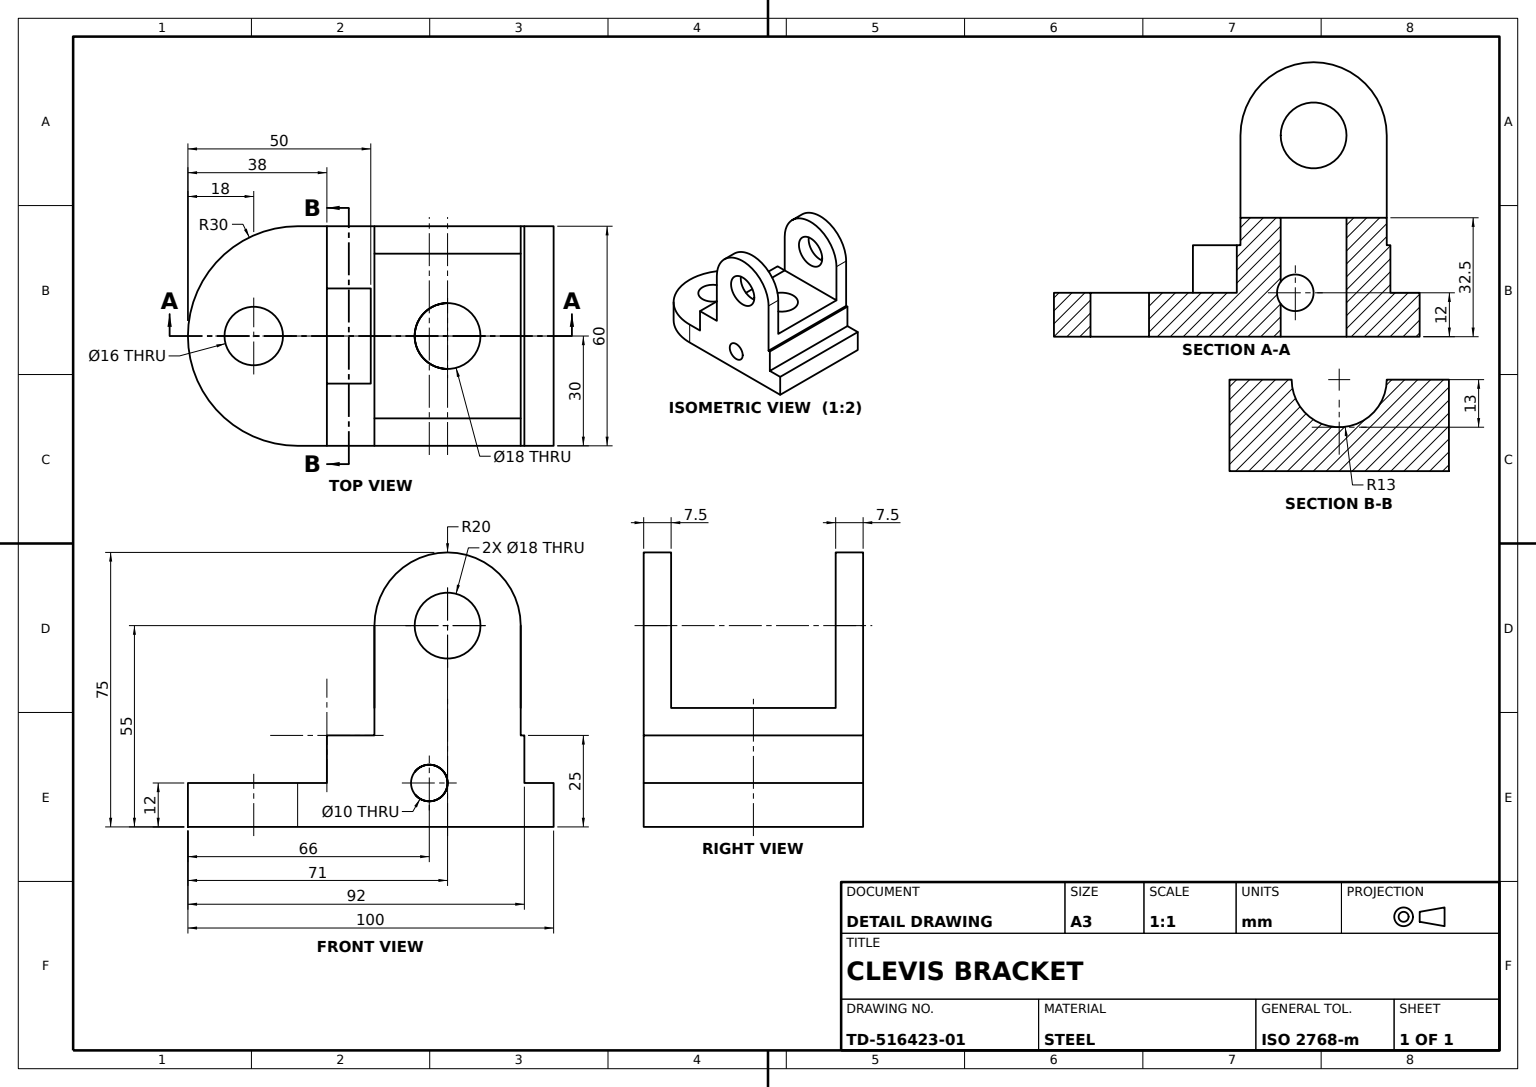
ISO-10303-21;
HEADER;
FILE_DESCRIPTION((''),'2;1');
FILE_NAME('','',(''),(''),'','','');
FILE_SCHEMA(('AUTOMOTIVE_DESIGN'));
ENDSEC;
DATA;
#1=APPLICATION_CONTEXT('');
#2=PRODUCT_CONTEXT('',#1,'mechanical');
#3=PRODUCT('','','',(#2));
#4=PRODUCT_DEFINITION_FORMATION('','',#3);
#5=PRODUCT_DEFINITION_CONTEXT('',#1,'design');
#6=PRODUCT_DEFINITION('','',#4,#5);
#7=PRODUCT_DEFINITION_SHAPE('','',#6);
#8=(LENGTH_UNIT()NAMED_UNIT(*)SI_UNIT(.MILLI.,.METRE.));
#9=(NAMED_UNIT(*)PLANE_ANGLE_UNIT()SI_UNIT($,.RADIAN.));
#10=(NAMED_UNIT(*)SI_UNIT($,.STERADIAN.)SOLID_ANGLE_UNIT());
#11=UNCERTAINTY_MEASURE_WITH_UNIT(LENGTH_MEASURE(1.E-05),#8,'distance_accuracy_value','');
#12=(GEOMETRIC_REPRESENTATION_CONTEXT(3)GLOBAL_UNCERTAINTY_ASSIGNED_CONTEXT((#11))GLOBAL_UNIT_ASSIGNED_CONTEXT((#8,#9,#10))REPRESENTATION_CONTEXT('',''));
#13=CARTESIAN_POINT('',(0.,0.,0.));
#14=VERTEX_POINT('',#13);
#15=CARTESIAN_POINT('',(30.,0.,-30.));
#16=VERTEX_POINT('',#15);
#17=CARTESIAN_POINT('',(0.,0.,-30.));
#18=DIRECTION('',(0.,1.,0.));
#19=DIRECTION('',(0.,0.,1.));
#20=AXIS2_PLACEMENT_3D('',#17,#18,#19);
#21=CIRCLE('',#20,30.);
#22=EDGE_CURVE('',#14,#16,#21,.T.);
#23=ORIENTED_EDGE('',*,*,#22,.T.);
#24=CARTESIAN_POINT('',(30.,12.,-30.));
#25=VERTEX_POINT('',#24);
#26=VECTOR('',#18,1000.);
#27=LINE('',#15,#26);
#28=EDGE_CURVE('',#16,#25,#27,.T.);
#29=ORIENTED_EDGE('',*,*,#28,.T.);
#30=CARTESIAN_POINT('',(0.,12.,0.));
#31=VERTEX_POINT('',#30);
#32=CARTESIAN_POINT('',(0.,12.,-30.));
#33=AXIS2_PLACEMENT_3D('',#32,#18,#19);
#34=CIRCLE('',#33,30.);
#35=EDGE_CURVE('',#31,#25,#34,.T.);
#36=ORIENTED_EDGE('',*,*,#35,.F.);
#37=LINE('',#13,#26);
#38=EDGE_CURVE('',#14,#31,#37,.T.);
#39=ORIENTED_EDGE('',*,*,#38,.F.);
#40=EDGE_LOOP('',(#23,#29,#36,#39));
#41=FACE_OUTER_BOUND('',#40,.T.);
#42=CYLINDRICAL_SURFACE('',#20,30.);
#43=ADVANCED_FACE('',(#41),#42,.T.);
#44=CARTESIAN_POINT('',(-22.5,55.,-51.));
#45=VERTEX_POINT('',#44);
#46=CARTESIAN_POINT('',(-30.,55.,-51.));
#47=VERTEX_POINT('',#46);
#48=DIRECTION('',(-1.,0.,0.));
#49=VECTOR('',#48,1000.);
#50=LINE('',#44,#49);
#51=EDGE_CURVE('',#45,#47,#50,.T.);
#52=ORIENTED_EDGE('',*,*,#51,.F.);
#53=CARTESIAN_POINT('',(-22.5,55.,-91.));
#54=VERTEX_POINT('',#53);
#55=CARTESIAN_POINT('',(-22.5,55.,-71.));
#56=AXIS2_PLACEMENT_3D('',#55,#48,#19);
#57=CIRCLE('',#56,20.);
#58=EDGE_CURVE('',#45,#54,#57,.T.);
#59=ORIENTED_EDGE('',*,*,#58,.T.);
#60=CARTESIAN_POINT('',(-30.,55.,-91.));
#61=VERTEX_POINT('',#60);
#62=LINE('',#53,#49);
#63=EDGE_CURVE('',#54,#61,#62,.T.);
#64=ORIENTED_EDGE('',*,*,#63,.T.);
#65=CARTESIAN_POINT('',(-30.,55.,-71.));
#66=AXIS2_PLACEMENT_3D('',#65,#48,#19);
#67=CIRCLE('',#66,20.);
#68=EDGE_CURVE('',#47,#61,#67,.T.);
#69=ORIENTED_EDGE('',*,*,#68,.F.);
#70=EDGE_LOOP('',(#52,#59,#64,#69));
#71=FACE_OUTER_BOUND('',#70,.T.);
#72=CYLINDRICAL_SURFACE('',#56,20.);
#73=ADVANCED_FACE('',(#71),#72,.T.);
#74=CARTESIAN_POINT('',(-9.,12.,-71.));
#75=VERTEX_POINT('',#74);
#76=CARTESIAN_POINT('',(-30.,12.,-71.));
#77=VERTEX_POINT('',#76);
#78=CARTESIAN_POINT('',(109.,12.,-71.));
#79=LINE('',#78,#49);
#80=EDGE_CURVE('',#75,#77,#79,.T.);
#81=ORIENTED_EDGE('',*,*,#80,.T.);
#82=CARTESIAN_POINT('',(-30.,12.,-61.));
#83=VERTEX_POINT('',#82);
#84=CARTESIAN_POINT('',(-30.,12.,-66.));
#85=AXIS2_PLACEMENT_3D('',#84,#48,#19);
#86=CIRCLE('',#85,5.);
#87=EDGE_CURVE('',#77,#83,#86,.T.);
#88=ORIENTED_EDGE('',*,*,#87,.T.);
#89=CARTESIAN_POINT('',(30.,12.,-61.));
#90=VERTEX_POINT('',#89);
#91=CARTESIAN_POINT('',(109.,12.,-61.));
#92=LINE('',#91,#49);
#93=EDGE_CURVE('',#90,#83,#92,.T.);
#94=ORIENTED_EDGE('',*,*,#93,.F.);
#95=CARTESIAN_POINT('',(30.,12.,-71.));
#96=VERTEX_POINT('',#95);
#97=CARTESIAN_POINT('',(30.,12.,-66.));
#98=AXIS2_PLACEMENT_3D('',#97,#48,#19);
#99=CIRCLE('',#98,5.);
#100=EDGE_CURVE('',#96,#90,#99,.T.);
#101=ORIENTED_EDGE('',*,*,#100,.F.);
#102=CARTESIAN_POINT('',(9.,12.,-71.));
#103=VERTEX_POINT('',#102);
#104=EDGE_CURVE('',#96,#103,#79,.T.);
#105=ORIENTED_EDGE('',*,*,#104,.T.);
#106=CARTESIAN_POINT('',(0.,9.,-62.));
#107=VERTEX_POINT('',#106);
#108=CARTESIAN_POINT('',(0.726741,9.,-62.));
#109=CARTESIAN_POINT('',(1.425372,8.878675,-62.086112));
#110=CARTESIAN_POINT('',(2.78525,8.507616,-62.413297));
#111=CARTESIAN_POINT('',(3.418337,8.271309,-62.647057));
#112=CARTESIAN_POINT('',(4.62738,7.806026,-63.251191));
#113=CARTESIAN_POINT('',(5.207095,7.573243,-63.626891));
#114=CARTESIAN_POINT('',(6.004777,7.296465,-64.287192));
#115=CARTESIAN_POINT('',(6.25998,7.215535,-64.524061));
#116=CARTESIAN_POINT('',(6.748974,7.08685,-65.035396));
#117=CARTESIAN_POINT('',(6.982797,7.039437,-65.310668));
#118=CARTESIAN_POINT('',(7.412294,6.993142,-65.882789));
#119=CARTESIAN_POINT('',(7.610136,6.993459,-66.181706));
#120=CARTESIAN_POINT('',(7.971358,7.055463,-66.806245));
#121=CARTESIAN_POINT('',(8.130031,7.11693,-67.124357));
#122=CARTESIAN_POINT('',(8.333866,7.259246,-67.597621));
#123=CARTESIAN_POINT('',(8.396386,7.315115,-67.755208));
#124=CARTESIAN_POINT('',(8.511134,7.445157,-68.069373));
#125=CARTESIAN_POINT('',(8.56369,7.519975,-68.22709));
#126=CARTESIAN_POINT('',(8.703959,7.769668,-68.688216));
#127=CARTESIAN_POINT('',(8.774291,7.968011,-68.978175));
#128=CARTESIAN_POINT('',(8.854745,8.314584,-69.383685));
#129=CARTESIAN_POINT('',(8.877469,8.439192,-69.51469));
#130=CARTESIAN_POINT('',(8.915274,8.701158,-69.761654));
#131=CARTESIAN_POINT('',(8.930378,8.83809,-69.877421));
#132=CARTESIAN_POINT('',(8.954911,9.123576,-70.093685));
#133=CARTESIAN_POINT('',(8.964335,9.27213,-70.194182));
#134=CARTESIAN_POINT('',(8.979072,9.58097,-70.379581));
#135=CARTESIAN_POINT('',(8.984396,9.742225,-70.46487));
#136=CARTESIAN_POINT('',(8.995994,10.234201,-70.691738));
#137=CARTESIAN_POINT('',(8.998241,10.574237,-70.805941));
#138=CARTESIAN_POINT('',(8.999745,11.10219,-70.922033));
#139=CARTESIAN_POINT('',(8.99989,11.282257,-70.951512));
#140=CARTESIAN_POINT('',(9.000016,11.641387,-70.990393));
#141=CARTESIAN_POINT('',(9.,11.820779,-71.));
#142=B_SPLINE_CURVE_WITH_KNOTS('',3,(#106,#108,#109,#110,#111,#112,#113,#114,#115,#116,#117,#118,#119,#120,#121,#122,#123,#124,#125,#126,#127,#128,#129,#130,#131,#132,#133,#134,#135,#136,#137,#138,#139,#140,#141,#102),.UNSPECIFIED.,.F.,.F.,(4,2,2,2,2,2,2,2,2,2,2,2,2,2,2,2,2,4),(0.,0.002142157,0.004284315,0.006426472,0.007497551,0.00856863,0.009639708,0.010710787,0.011246327,0.011781866,0.012852945,0.013388484,0.013924023,0.014459563,0.014995102,0.016066181,0.01660172,0.01713726),.UNSPECIFIED.);
#143=EDGE_CURVE('',#107,#103,#142,.T.);
#144=ORIENTED_EDGE('',*,*,#143,.F.);
#145=CARTESIAN_POINT('',(-9.,11.8209,-71.));
#146=CARTESIAN_POINT('',(-9.000016,11.641774,-70.990405));
#147=CARTESIAN_POINT('',(-8.999891,11.283468,-70.951672));
#148=CARTESIAN_POINT('',(-8.999747,11.103386,-70.922255));
#149=CARTESIAN_POINT('',(-8.998246,10.575033,-70.806197));
#150=CARTESIAN_POINT('',(-8.995995,10.235538,-70.692133));
#151=CARTESIAN_POINT('',(-8.984485,9.745344,-70.466417));
#152=CARTESIAN_POINT('',(-8.979195,9.584172,-70.381362));
#153=CARTESIAN_POINT('',(-8.964482,9.274613,-70.195811));
#154=CARTESIAN_POINT('',(-8.955082,9.126074,-70.095418));
#155=CARTESIAN_POINT('',(-8.93069,8.841205,-69.879937));
#156=CARTESIAN_POINT('',(-8.915701,8.704875,-69.764847));
#157=CARTESIAN_POINT('',(-8.878347,8.444548,-69.520041));
#158=CARTESIAN_POINT('',(-8.855808,8.319832,-69.389454));
#159=CARTESIAN_POINT('',(-8.775159,7.970443,-68.981745));
#160=CARTESIAN_POINT('',(-8.704837,7.772204,-68.691882));
#161=CARTESIAN_POINT('',(-8.519744,7.440793,-68.081856));
#162=CARTESIAN_POINT('',(-8.403721,7.308286,-67.760082));
#163=CARTESIAN_POINT('',(-8.198666,7.164719,-67.283581));
#164=CARTESIAN_POINT('',(-8.124892,7.125469,-67.124746));
#165=CARTESIAN_POINT('',(-7.965912,7.063018,-66.807662));
#166=CARTESIAN_POINT('',(-7.880201,7.03977,-66.648579));
#167=CARTESIAN_POINT('',(-7.609601,6.99346,-66.1809));
#168=CARTESIAN_POINT('',(-7.411303,6.993087,-65.881207));
#169=CARTESIAN_POINT('',(-6.979026,7.040007,-65.305911));
#170=CARTESIAN_POINT('',(-6.745093,7.087759,-65.031095));
#171=CARTESIAN_POINT('',(-6.257885,7.216199,-64.522116));
#172=CARTESIAN_POINT('',(-6.002691,7.29713,-64.285268));
#173=CARTESIAN_POINT('',(-5.468957,7.482442,-63.843853));
#174=CARTESIAN_POINT('',(-5.188651,7.587613,-63.638291));
#175=CARTESIAN_POINT('',(-4.61524,7.808165,-63.265892));
#176=CARTESIAN_POINT('',(-4.321594,7.92372,-63.098261));
#177=CARTESIAN_POINT('',(-3.718366,8.15583,-62.79711));
#178=CARTESIAN_POINT('',(-3.408815,8.272473,-62.663595));
#179=CARTESIAN_POINT('',(-2.769917,8.495453,-62.430097));
#180=CARTESIAN_POINT('',(-2.437965,8.602548,-62.329528));
#181=CARTESIAN_POINT('',(-1.762154,8.786606,-62.167358));
#182=CARTESIAN_POINT('',(-1.419129,8.863377,-62.10562));
#183=CARTESIAN_POINT('',(-0.720045,8.970201,-62.021945));
#184=CARTESIAN_POINT('',(-0.362595,9.,-62.));
#185=B_SPLINE_CURVE_WITH_KNOTS('',3,(#74,#145,#146,#147,#148,#149,#150,#151,#152,#153,#154,#155,#156,#157,#158,#159,#160,#161,#162,#163,#164,#165,#166,#167,#168,#169,#170,#171,#172,#173,#174,#175,#176,#177,#178,#179,#180,#181,#182,#183,#184,#106),.UNSPECIFIED.,.F.,.F.,(4,2,2,2,2,2,2,2,2,2,2,2,2,2,2,2,2,2,2,2,4),(0.051380768,0.051915165,0.052449561,0.053518354,0.054052751,0.054587147,0.055121544,0.05565594,0.056724733,0.057793526,0.058327923,0.058862319,0.059931112,0.060999905,0.062068698,0.063137491,0.064206284,0.065275077,0.06634387,0.067412663,0.068481455),.UNSPECIFIED.);
#186=EDGE_CURVE('',#75,#107,#185,.T.);
#187=ORIENTED_EDGE('',*,*,#186,.F.);
#188=EDGE_LOOP('',(#81,#88,#94,#101,#105,#144,#187));
#189=FACE_OUTER_BOUND('',#188,.T.);
#190=CARTESIAN_POINT('',(109.,12.,-66.));
#191=AXIS2_PLACEMENT_3D('',#190,#48,#19);
#192=CYLINDRICAL_SURFACE('',#191,5.);
#193=ADVANCED_FACE('',(#189),#192,.F.);
#194=CARTESIAN_POINT('',(0.,12.,-38.));
#195=VERTEX_POINT('',#194);
#196=CARTESIAN_POINT('',(13.,25.,-38.));
#197=VERTEX_POINT('',#196);
#198=CARTESIAN_POINT('',(0.,25.,-38.));
#199=DIRECTION('',(1.,0.,0.));
#200=AXIS2_PLACEMENT_3D('',#198,#19,#199);
#201=CIRCLE('',#200,13.);
#202=EDGE_CURVE('',#195,#197,#201,.T.);
#203=ORIENTED_EDGE('',*,*,#202,.F.);
#204=CARTESIAN_POINT('',(30.,12.,-38.));
#205=VERTEX_POINT('',#204);
#206=CARTESIAN_POINT('',(-30.,12.,-38.));
#207=VECTOR('',#199,1000.);
#208=LINE('',#206,#207);
#209=EDGE_CURVE('',#195,#205,#208,.T.);
#210=ORIENTED_EDGE('',*,*,#209,.T.);
#211=CARTESIAN_POINT('',(30.,25.,-38.));
#212=VERTEX_POINT('',#211);
#213=DIRECTION('',(0.,-1.,0.));
#214=VECTOR('',#213,1000.);
#215=LINE('',#204,#214);
#216=EDGE_CURVE('',#212,#205,#215,.T.);
#217=ORIENTED_EDGE('',*,*,#216,.F.);
#218=CARTESIAN_POINT('',(-30.,25.,-38.));
#219=LINE('',#218,#207);
#220=EDGE_CURVE('',#197,#212,#219,.T.);
#221=ORIENTED_EDGE('',*,*,#220,.F.);
#222=EDGE_LOOP('',(#203,#210,#217,#221));
#223=FACE_OUTER_BOUND('',#222,.T.);
#224=AXIS2_PLACEMENT_3D('',#206,#19,#199);
#225=PLANE('',#224);
#226=ADVANCED_FACE('',(#223),#225,.T.);
#227=CARTESIAN_POINT('',(30.,12.,-100.));
#228=VERTEX_POINT('',#227);
#229=CARTESIAN_POINT('',(-30.,12.,-100.));
#230=VERTEX_POINT('',#229);
#231=LINE('',#229,#49);
#232=EDGE_CURVE('',#228,#230,#231,.T.);
#233=ORIENTED_EDGE('',*,*,#232,.F.);
#234=CARTESIAN_POINT('',(30.,0.,-100.));
#235=VERTEX_POINT('',#234);
#236=LINE('',#227,#214);
#237=EDGE_CURVE('',#228,#235,#236,.T.);
#238=ORIENTED_EDGE('',*,*,#237,.T.);
#239=CARTESIAN_POINT('',(-30.,0.,-100.));
#240=VERTEX_POINT('',#239);
#241=LINE('',#239,#49);
#242=EDGE_CURVE('',#235,#240,#241,.T.);
#243=ORIENTED_EDGE('',*,*,#242,.T.);
#244=LINE('',#229,#214);
#245=EDGE_CURVE('',#230,#240,#244,.T.);
#246=ORIENTED_EDGE('',*,*,#245,.F.);
#247=EDGE_LOOP('',(#233,#238,#243,#246));
#248=FACE_OUTER_BOUND('',#247,.T.);
#249=AXIS2_PLACEMENT_3D('',#229,#19,#199);
#250=PLANE('',#249);
#251=ADVANCED_FACE('',(#248),#250,.F.);
#252=CARTESIAN_POINT('',(-30.,25.,-91.));
#253=VERTEX_POINT('',#252);
#254=CARTESIAN_POINT('',(-30.,25.,-92.));
#255=VERTEX_POINT('',#254);
#256=CARTESIAN_POINT('',(-30.,25.,0.));
#257=DIRECTION('',(0.,0.,-1.));
#258=VECTOR('',#257,1000.);
#259=LINE('',#256,#258);
#260=EDGE_CURVE('',#253,#255,#259,.T.);
#261=ORIENTED_EDGE('',*,*,#260,.F.);
#262=CARTESIAN_POINT('',(30.,25.,-91.));
#263=VERTEX_POINT('',#262);
#264=CARTESIAN_POINT('',(-22.5,25.,-91.));
#265=LINE('',#264,#49);
#266=EDGE_CURVE('',#263,#253,#265,.T.);
#267=ORIENTED_EDGE('',*,*,#266,.F.);
#268=CARTESIAN_POINT('',(30.,25.,-92.));
#269=VERTEX_POINT('',#268);
#270=CARTESIAN_POINT('',(30.,25.,0.));
#271=LINE('',#270,#258);
#272=EDGE_CURVE('',#263,#269,#271,.T.);
#273=ORIENTED_EDGE('',*,*,#272,.T.);
#274=LINE('',#254,#207);
#275=EDGE_CURVE('',#255,#269,#274,.T.);
#276=ORIENTED_EDGE('',*,*,#275,.F.);
#277=EDGE_LOOP('',(#261,#267,#273,#276));
#278=FACE_OUTER_BOUND('',#277,.T.);
#279=AXIS2_PLACEMENT_3D('',#256,#213,#257);
#280=PLANE('',#279);
#281=ADVANCED_FACE('',(#278),#280,.F.);
#282=CARTESIAN_POINT('',(22.5,55.,-51.));
#283=VERTEX_POINT('',#282);
#284=CARTESIAN_POINT('',(30.,55.,-51.));
#285=VERTEX_POINT('',#284);
#286=LINE('',#282,#207);
#287=EDGE_CURVE('',#283,#285,#286,.T.);
#288=ORIENTED_EDGE('',*,*,#287,.F.);
#289=CARTESIAN_POINT('',(22.5,32.5,-51.));
#290=VERTEX_POINT('',#289);
#291=LINE('',#282,#26);
#292=EDGE_CURVE('',#290,#283,#291,.T.);
#293=ORIENTED_EDGE('',*,*,#292,.F.);
#294=CARTESIAN_POINT('',(-22.5,32.5,-51.));
#295=VERTEX_POINT('',#294);
#296=LINE('',#294,#207);
#297=EDGE_CURVE('',#295,#290,#296,.T.);
#298=ORIENTED_EDGE('',*,*,#297,.F.);
#299=LINE('',#44,#26);
#300=EDGE_CURVE('',#295,#45,#299,.T.);
#301=ORIENTED_EDGE('',*,*,#300,.T.);
#302=ORIENTED_EDGE('',*,*,#51,.T.);
#303=CARTESIAN_POINT('',(-30.,25.,-51.));
#304=VERTEX_POINT('',#303);
#305=LINE('',#46,#26);
#306=EDGE_CURVE('',#304,#47,#305,.T.);
#307=ORIENTED_EDGE('',*,*,#306,.F.);
#308=CARTESIAN_POINT('',(30.,25.,-51.));
#309=VERTEX_POINT('',#308);
#310=CARTESIAN_POINT('',(-22.5,25.,-51.));
#311=LINE('',#310,#49);
#312=EDGE_CURVE('',#309,#304,#311,.T.);
#313=ORIENTED_EDGE('',*,*,#312,.F.);
#314=LINE('',#284,#26);
#315=EDGE_CURVE('',#309,#285,#314,.T.);
#316=ORIENTED_EDGE('',*,*,#315,.T.);
#317=EDGE_LOOP('',(#288,#293,#298,#301,#302,#307,#313,#316));
#318=FACE_OUTER_BOUND('',#317,.T.);
#319=AXIS2_PLACEMENT_3D('',#44,#19,#199);
#320=PLANE('',#319);
#321=ADVANCED_FACE('',(#318),#320,.T.);
#322=CARTESIAN_POINT('',(-30.,0.,-30.));
#323=VERTEX_POINT('',#322);
#324=CARTESIAN_POINT('',(-30.,12.,-30.));
#325=VERTEX_POINT('',#324);
#326=LINE('',#322,#26);
#327=EDGE_CURVE('',#323,#325,#326,.T.);
#328=ORIENTED_EDGE('',*,*,#327,.F.);
#329=EDGE_CURVE('',#323,#14,#21,.T.);
#330=ORIENTED_EDGE('',*,*,#329,.T.);
#331=ORIENTED_EDGE('',*,*,#38,.T.);
#332=EDGE_CURVE('',#325,#31,#34,.T.);
#333=ORIENTED_EDGE('',*,*,#332,.F.);
#334=EDGE_LOOP('',(#328,#330,#331,#333));
#335=FACE_OUTER_BOUND('',#334,.T.);
#336=ADVANCED_FACE('',(#335),#42,.T.);
#337=CARTESIAN_POINT('',(30.,12.,-92.));
#338=VERTEX_POINT('',#337);
#339=LINE('',#227,#258);
#340=EDGE_CURVE('',#338,#228,#339,.T.);
#341=ORIENTED_EDGE('',*,*,#340,.T.);
#342=ORIENTED_EDGE('',*,*,#232,.T.);
#343=CARTESIAN_POINT('',(-30.,12.,-92.));
#344=VERTEX_POINT('',#343);
#345=CARTESIAN_POINT('',(-30.,12.,0.));
#346=VECTOR('',#19,1000.);
#347=LINE('',#345,#346);
#348=EDGE_CURVE('',#230,#344,#347,.T.);
#349=ORIENTED_EDGE('',*,*,#348,.T.);
#350=CARTESIAN_POINT('',(0.,12.,-92.));
#351=LINE('',#350,#49);
#352=EDGE_CURVE('',#338,#344,#351,.T.);
#353=ORIENTED_EDGE('',*,*,#352,.F.);
#354=EDGE_LOOP('',(#341,#342,#349,#353));
#355=FACE_OUTER_BOUND('',#354,.T.);
#356=AXIS2_PLACEMENT_3D('',#30,#213,#257);
#357=PLANE('',#356);
#358=ADVANCED_FACE('',(#355),#357,.F.);
#359=CARTESIAN_POINT('',(-22.5,55.,-62.));
#360=VERTEX_POINT('',#359);
#361=CARTESIAN_POINT('',(-30.,55.,-62.));
#362=VERTEX_POINT('',#361);
#363=CARTESIAN_POINT('',(109.,55.,-62.));
#364=LINE('',#363,#49);
#365=EDGE_CURVE('',#360,#362,#364,.T.);
#366=ORIENTED_EDGE('',*,*,#365,.F.);
#367=CARTESIAN_POINT('',(-22.5,55.,-80.));
#368=VERTEX_POINT('',#367);
#369=CIRCLE('',#56,9.);
#370=EDGE_CURVE('',#368,#360,#369,.T.);
#371=ORIENTED_EDGE('',*,*,#370,.F.);
#372=CARTESIAN_POINT('',(-30.,55.,-80.));
#373=VERTEX_POINT('',#372);
#374=CARTESIAN_POINT('',(109.,55.,-80.));
#375=LINE('',#374,#49);
#376=EDGE_CURVE('',#368,#373,#375,.T.);
#377=ORIENTED_EDGE('',*,*,#376,.T.);
#378=CIRCLE('',#66,9.);
#379=EDGE_CURVE('',#373,#362,#378,.T.);
#380=ORIENTED_EDGE('',*,*,#379,.T.);
#381=EDGE_LOOP('',(#366,#371,#377,#380));
#382=FACE_OUTER_BOUND('',#381,.T.);
#383=CARTESIAN_POINT('',(109.,55.,-71.));
#384=AXIS2_PLACEMENT_3D('',#383,#48,#19);
#385=CYLINDRICAL_SURFACE('',#384,9.);
#386=ADVANCED_FACE('',(#382),#385,.F.);
#387=CARTESIAN_POINT('',(0.,0.,-10.));
#388=VERTEX_POINT('',#387);
#389=CARTESIAN_POINT('',(0.,0.,-26.));
#390=VERTEX_POINT('',#389);
#391=CARTESIAN_POINT('',(0.,0.,-18.));
#392=AXIS2_PLACEMENT_3D('',#391,#213,#257);
#393=CIRCLE('',#392,8.);
#394=EDGE_CURVE('',#388,#390,#393,.T.);
#395=ORIENTED_EDGE('',*,*,#394,.T.);
#396=CARTESIAN_POINT('',(0.,12.,-26.));
#397=VERTEX_POINT('',#396);
#398=CARTESIAN_POINT('',(0.,-127.,-26.));
#399=LINE('',#398,#26);
#400=EDGE_CURVE('',#390,#397,#399,.T.);
#401=ORIENTED_EDGE('',*,*,#400,.T.);
#402=CARTESIAN_POINT('',(0.,12.,-10.));
#403=VERTEX_POINT('',#402);
#404=CARTESIAN_POINT('',(0.,12.,-18.));
#405=AXIS2_PLACEMENT_3D('',#404,#18,#19);
#406=CIRCLE('',#405,8.);
#407=EDGE_CURVE('',#397,#403,#406,.T.);
#408=ORIENTED_EDGE('',*,*,#407,.T.);
#409=CARTESIAN_POINT('',(0.,-127.,-10.));
#410=LINE('',#409,#26);
#411=EDGE_CURVE('',#388,#403,#410,.T.);
#412=ORIENTED_EDGE('',*,*,#411,.F.);
#413=EDGE_LOOP('',(#395,#401,#408,#412));
#414=FACE_OUTER_BOUND('',#413,.T.);
#415=CARTESIAN_POINT('',(0.,-127.,-18.));
#416=AXIS2_PLACEMENT_3D('',#415,#18,#19);
#417=CYLINDRICAL_SURFACE('',#416,8.);
#418=ADVANCED_FACE('',(#414),#417,.F.);
#419=ORIENTED_EDGE('',*,*,#352,.T.);
#420=CARTESIAN_POINT('',(-30.,0.,-92.));
#421=LINE('',#420,#214);
#422=EDGE_CURVE('',#255,#344,#421,.T.);
#423=ORIENTED_EDGE('',*,*,#422,.F.);
#424=ORIENTED_EDGE('',*,*,#275,.T.);
#425=CARTESIAN_POINT('',(30.,0.,-92.));
#426=LINE('',#425,#214);
#427=EDGE_CURVE('',#269,#338,#426,.T.);
#428=ORIENTED_EDGE('',*,*,#427,.T.);
#429=EDGE_LOOP('',(#419,#423,#424,#428));
#430=FACE_OUTER_BOUND('',#429,.T.);
#431=AXIS2_PLACEMENT_3D('',#420,#19,#199);
#432=PLANE('',#431);
#433=ADVANCED_FACE('',(#430),#432,.F.);
#434=EDGE_CURVE('',#403,#397,#406,.T.);
#435=ORIENTED_EDGE('',*,*,#434,.T.);
#436=ORIENTED_EDGE('',*,*,#400,.F.);
#437=EDGE_CURVE('',#390,#388,#393,.T.);
#438=ORIENTED_EDGE('',*,*,#437,.T.);
#439=ORIENTED_EDGE('',*,*,#411,.T.);
#440=EDGE_LOOP('',(#435,#436,#438,#439));
#441=FACE_OUTER_BOUND('',#440,.T.);
#442=ADVANCED_FACE('',(#441),#417,.F.);
#443=ORIENTED_EDGE('',*,*,#370,.T.);
#444=EDGE_CURVE('',#360,#368,#369,.T.);
#445=ORIENTED_EDGE('',*,*,#444,.T.);
#446=EDGE_LOOP('',(#443,#445));
#447=FACE_BOUND('',#446,.T.);
#448=CARTESIAN_POINT('',(-22.5,32.5,-91.));
#449=VERTEX_POINT('',#448);
#450=LINE('',#264,#214);
#451=EDGE_CURVE('',#54,#449,#450,.T.);
#452=ORIENTED_EDGE('',*,*,#451,.F.);
#453=ORIENTED_EDGE('',*,*,#58,.F.);
#454=ORIENTED_EDGE('',*,*,#300,.F.);
#455=LINE('',#448,#346);
#456=EDGE_CURVE('',#449,#295,#455,.T.);
#457=ORIENTED_EDGE('',*,*,#456,.F.);
#458=EDGE_LOOP('',(#452,#453,#454,#457));
#459=FACE_OUTER_BOUND('',#458,.T.);
#460=PLANE('',#56);
#461=ADVANCED_FACE('',(#447,#459),#460,.F.);
#462=ORIENTED_EDGE('',*,*,#100,.T.);
#463=EDGE_CURVE('',#90,#96,#99,.T.);
#464=ORIENTED_EDGE('',*,*,#463,.T.);
#465=EDGE_LOOP('',(#462,#464));
#466=FACE_BOUND('',#465,.T.);
#467=CARTESIAN_POINT('',(30.,55.,-62.));
#468=VERTEX_POINT('',#467);
#469=CARTESIAN_POINT('',(30.,55.,-80.));
#470=VERTEX_POINT('',#469);
#471=CARTESIAN_POINT('',(30.,55.,-71.));
#472=AXIS2_PLACEMENT_3D('',#471,#48,#19);
#473=CIRCLE('',#472,9.);
#474=EDGE_CURVE('',#468,#470,#473,.T.);
#475=ORIENTED_EDGE('',*,*,#474,.T.);
#476=EDGE_CURVE('',#470,#468,#473,.T.);
#477=ORIENTED_EDGE('',*,*,#476,.T.);
#478=EDGE_LOOP('',(#475,#477));
#479=FACE_BOUND('',#478,.T.);
#480=EDGE_CURVE('',#212,#309,#271,.T.);
#481=ORIENTED_EDGE('',*,*,#480,.F.);
#482=ORIENTED_EDGE('',*,*,#216,.T.);
#483=EDGE_CURVE('',#25,#205,#339,.T.);
#484=ORIENTED_EDGE('',*,*,#483,.F.);
#485=ORIENTED_EDGE('',*,*,#28,.F.);
#486=LINE('',#234,#258);
#487=EDGE_CURVE('',#16,#235,#486,.T.);
#488=ORIENTED_EDGE('',*,*,#487,.T.);
#489=ORIENTED_EDGE('',*,*,#237,.F.);
#490=ORIENTED_EDGE('',*,*,#340,.F.);
#491=ORIENTED_EDGE('',*,*,#427,.F.);
#492=ORIENTED_EDGE('',*,*,#272,.F.);
#493=CARTESIAN_POINT('',(30.,55.,-91.));
#494=VERTEX_POINT('',#493);
#495=LINE('',#262,#214);
#496=EDGE_CURVE('',#494,#263,#495,.T.);
#497=ORIENTED_EDGE('',*,*,#496,.F.);
#498=CIRCLE('',#472,20.);
#499=EDGE_CURVE('',#285,#494,#498,.T.);
#500=ORIENTED_EDGE('',*,*,#499,.F.);
#501=ORIENTED_EDGE('',*,*,#315,.F.);
#502=EDGE_LOOP('',(#481,#482,#484,#485,#488,#489,#490,#491,#492,#497,#500,#501));
#503=FACE_OUTER_BOUND('',#502,.T.);
#504=AXIS2_PLACEMENT_3D('',#227,#48,#19);
#505=PLANE('',#504);
#506=ADVANCED_FACE('',(#466,#479,#503),#505,.F.);
#507=ORIENTED_EDGE('',*,*,#407,.F.);
#508=ORIENTED_EDGE('',*,*,#434,.F.);
#509=EDGE_LOOP('',(#507,#508));
#510=FACE_BOUND('',#509,.T.);
#511=ORIENTED_EDGE('',*,*,#35,.T.);
#512=ORIENTED_EDGE('',*,*,#483,.T.);
#513=ORIENTED_EDGE('',*,*,#209,.F.);
#514=VERTEX_POINT('',#206);
#515=EDGE_CURVE('',#514,#195,#208,.T.);
#516=ORIENTED_EDGE('',*,*,#515,.F.);
#517=EDGE_CURVE('',#514,#325,#347,.T.);
#518=ORIENTED_EDGE('',*,*,#517,.T.);
#519=ORIENTED_EDGE('',*,*,#332,.T.);
#520=EDGE_LOOP('',(#511,#512,#513,#516,#518,#519));
#521=FACE_OUTER_BOUND('',#520,.T.);
#522=ADVANCED_FACE('',(#510,#521),#357,.F.);
#523=ORIENTED_EDGE('',*,*,#476,.F.);
#524=CARTESIAN_POINT('',(22.5,55.,-80.));
#525=VERTEX_POINT('',#524);
#526=EDGE_CURVE('',#470,#525,#375,.T.);
#527=ORIENTED_EDGE('',*,*,#526,.T.);
#528=CARTESIAN_POINT('',(22.5,55.,-62.));
#529=VERTEX_POINT('',#528);
#530=CARTESIAN_POINT('',(22.5,55.,-71.));
#531=AXIS2_PLACEMENT_3D('',#530,#199,#257);
#532=CIRCLE('',#531,9.);
#533=EDGE_CURVE('',#529,#525,#532,.T.);
#534=ORIENTED_EDGE('',*,*,#533,.F.);
#535=EDGE_CURVE('',#468,#529,#364,.T.);
#536=ORIENTED_EDGE('',*,*,#535,.F.);
#537=EDGE_LOOP('',(#523,#527,#534,#536));
#538=FACE_OUTER_BOUND('',#537,.T.);
#539=ADVANCED_FACE('',(#538),#385,.F.);
#540=CARTESIAN_POINT('',(22.5,32.5,-91.));
#541=VERTEX_POINT('',#540);
#542=LINE('',#289,#258);
#543=EDGE_CURVE('',#290,#541,#542,.T.);
#544=ORIENTED_EDGE('',*,*,#543,.T.);
#545=LINE('',#540,#49);
#546=EDGE_CURVE('',#541,#449,#545,.T.);
#547=ORIENTED_EDGE('',*,*,#546,.T.);
#548=ORIENTED_EDGE('',*,*,#456,.T.);
#549=ORIENTED_EDGE('',*,*,#297,.T.);
#550=EDGE_LOOP('',(#544,#547,#548,#549));
#551=FACE_OUTER_BOUND('',#550,.T.);
#552=CARTESIAN_POINT('',(0.,32.5,-80.));
#553=VERTEX_POINT('',#552);
#554=CARTESIAN_POINT('',(0.,32.5,-62.));
#555=VERTEX_POINT('',#554);
#556=CARTESIAN_POINT('',(0.,32.5,-71.));
#557=AXIS2_PLACEMENT_3D('',#556,#18,#19);
#558=CIRCLE('',#557,9.);
#559=EDGE_CURVE('',#553,#555,#558,.T.);
#560=ORIENTED_EDGE('',*,*,#559,.F.);
#561=EDGE_CURVE('',#555,#553,#558,.T.);
#562=ORIENTED_EDGE('',*,*,#561,.F.);
#563=EDGE_LOOP('',(#560,#562));
#564=FACE_BOUND('',#563,.T.);
#565=CARTESIAN_POINT('',(0.,32.5,0.));
#566=AXIS2_PLACEMENT_3D('',#565,#18,#19);
#567=PLANE('',#566);
#568=ADVANCED_FACE('',(#551,#564),#567,.T.);
#569=VERTEX_POINT('',#218);
#570=CARTESIAN_POINT('',(-13.,25.,-38.));
#571=VERTEX_POINT('',#570);
#572=EDGE_CURVE('',#569,#571,#219,.T.);
#573=ORIENTED_EDGE('',*,*,#572,.F.);
#574=LINE('',#206,#214);
#575=EDGE_CURVE('',#569,#514,#574,.T.);
#576=ORIENTED_EDGE('',*,*,#575,.T.);
#577=ORIENTED_EDGE('',*,*,#515,.T.);
#578=EDGE_CURVE('',#571,#195,#201,.T.);
#579=ORIENTED_EDGE('',*,*,#578,.F.);
#580=EDGE_LOOP('',(#573,#576,#577,#579));
#581=FACE_OUTER_BOUND('',#580,.T.);
#582=ADVANCED_FACE('',(#581),#225,.T.);
#583=ORIENTED_EDGE('',*,*,#496,.T.);
#584=ORIENTED_EDGE('',*,*,#266,.T.);
#585=LINE('',#252,#214);
#586=EDGE_CURVE('',#61,#253,#585,.T.);
#587=ORIENTED_EDGE('',*,*,#586,.F.);
#588=ORIENTED_EDGE('',*,*,#63,.F.);
#589=ORIENTED_EDGE('',*,*,#451,.T.);
#590=ORIENTED_EDGE('',*,*,#546,.F.);
#591=CARTESIAN_POINT('',(22.5,55.,-91.));
#592=VERTEX_POINT('',#591);
#593=CARTESIAN_POINT('',(22.5,25.,-91.));
#594=LINE('',#593,#214);
#595=EDGE_CURVE('',#592,#541,#594,.T.);
#596=ORIENTED_EDGE('',*,*,#595,.F.);
#597=LINE('',#591,#207);
#598=EDGE_CURVE('',#592,#494,#597,.T.);
#599=ORIENTED_EDGE('',*,*,#598,.T.);
#600=EDGE_LOOP('',(#583,#584,#587,#588,#589,#590,#596,#599));
#601=FACE_OUTER_BOUND('',#600,.T.);
#602=AXIS2_PLACEMENT_3D('',#264,#257,#48);
#603=PLANE('',#602);
#604=ADVANCED_FACE('',(#601),#603,.T.);
#605=CARTESIAN_POINT('',(0.,15.,-62.));
#606=VERTEX_POINT('',#605);
#607=CARTESIAN_POINT('',(-0.36027,15.,-62.));
#608=CARTESIAN_POINT('',(-0.715709,15.029261,-62.021533));
#609=CARTESIAN_POINT('',(-1.418151,15.13635,-62.105397));
#610=CARTESIAN_POINT('',(-1.767872,15.214765,-62.168499));
#611=CARTESIAN_POINT('',(-2.781569,15.49141,-62.412449));
#612=CARTESIAN_POINT('',(-3.414457,15.727207,-62.645191));
#613=CARTESIAN_POINT('',(-4.325893,16.077946,-63.100507));
#614=CARTESIAN_POINT('',(-4.623435,16.195028,-63.270853));
#615=CARTESIAN_POINT('',(-5.194042,16.414419,-63.642161));
#616=CARTESIAN_POINT('',(-5.468826,16.517471,-63.843882));
#617=CARTESIAN_POINT('',(-5.998577,16.701483,-64.281729));
#618=CARTESIAN_POINT('',(-6.253537,16.782541,-64.51782));
#619=CARTESIAN_POINT('',(-6.743494,16.911931,-65.029182));
#620=CARTESIAN_POINT('',(-6.977499,16.959656,-65.304158));
#621=CARTESIAN_POINT('',(-7.407801,17.006703,-65.87627));
#622=CARTESIAN_POINT('',(-7.606326,17.006822,-66.175595));
#623=CARTESIAN_POINT('',(-7.969276,16.945262,-66.802176));
#624=CARTESIAN_POINT('',(-8.127177,16.884483,-67.118319));
#625=CARTESIAN_POINT('',(-8.331705,16.742545,-67.592317));
#626=CARTESIAN_POINT('',(-8.394517,16.686728,-67.750341));
#627=CARTESIAN_POINT('',(-8.509907,16.5565,-68.065773));
#628=CARTESIAN_POINT('',(-8.562735,16.481465,-68.224159));
#629=CARTESIAN_POINT('',(-8.702927,16.23268,-68.684413));
#630=CARTESIAN_POINT('',(-8.773514,16.034656,-68.974677));
#631=CARTESIAN_POINT('',(-8.854359,15.687418,-69.381528));
#632=CARTESIAN_POINT('',(-8.877191,15.562424,-69.513039));
#633=CARTESIAN_POINT('',(-8.91501,15.300973,-69.759772));
#634=CARTESIAN_POINT('',(-8.93015,15.164165,-69.875587));
#635=CARTESIAN_POINT('',(-8.954759,14.878595,-70.092164));
#636=CARTESIAN_POINT('',(-8.964226,14.729833,-70.192927));
#637=CARTESIAN_POINT('',(-8.979033,14.420168,-70.378974));
#638=CARTESIAN_POINT('',(-8.984365,14.258757,-70.464364));
#639=CARTESIAN_POINT('',(-8.99597,13.767433,-70.691089));
#640=CARTESIAN_POINT('',(-8.998236,13.427147,-70.805614));
#641=CARTESIAN_POINT('',(-8.999747,12.89757,-70.922097));
#642=CARTESIAN_POINT('',(-8.999891,12.717297,-70.951567));
#643=CARTESIAN_POINT('',(-9.000016,12.358689,-70.990378));
#644=CARTESIAN_POINT('',(-9.,12.179358,-71.));
#645=B_SPLINE_CURVE_WITH_KNOTS('',3,(#605,#607,#608,#609,#610,#611,#612,#613,#614,#615,#616,#617,#618,#619,#620,#621,#622,#623,#624,#625,#626,#627,#628,#629,#630,#631,#632,#633,#634,#635,#636,#637,#638,#639,#640,#641,#642,#643,#644,#74),.UNSPECIFIED.,.F.,.F.,(4,2,2,2,2,2,2,2,2,2,2,2,2,2,2,2,2,2,2,4),(0.034255444,0.035325777,0.03639611,0.038536775,0.039607108,0.040677441,0.041747773,0.042818106,0.043888439,0.044958772,0.045493938,0.046029105,0.047099437,0.047634604,0.04816977,0.048704936,0.049240103,0.050310436,0.050845602,0.051380768),.UNSPECIFIED.);
#646=EDGE_CURVE('',#606,#75,#645,.T.);
#647=ORIENTED_EDGE('',*,*,#646,.F.);
#648=CARTESIAN_POINT('',(9.,12.179022,-71.));
#649=CARTESIAN_POINT('',(9.000016,12.357874,-70.990413));
#650=CARTESIAN_POINT('',(8.999892,12.715235,-70.951842));
#651=CARTESIAN_POINT('',(8.99975,12.894805,-70.922599));
#652=CARTESIAN_POINT('',(8.998252,13.424319,-70.806446));
#653=CARTESIAN_POINT('',(8.995994,13.763739,-70.692338));
#654=CARTESIAN_POINT('',(8.980718,14.415844,-70.392324));
#655=CARTESIAN_POINT('',(8.967368,14.729907,-70.204193));
#656=CARTESIAN_POINT('',(8.918653,15.299899,-69.773366));
#657=CARTESIAN_POINT('',(8.883296,15.560334,-69.528877));
#658=CARTESIAN_POINT('',(8.775671,16.028079,-68.983879));
#659=CARTESIAN_POINT('',(8.705344,16.226451,-68.693903));
#660=CARTESIAN_POINT('',(8.520899,16.557572,-68.085316));
#661=CARTESIAN_POINT('',(8.405046,16.690435,-67.763517));
#662=CARTESIAN_POINT('',(8.13188,16.882388,-67.128032));
#663=CARTESIAN_POINT('',(7.973085,16.94401,-66.809524));
#664=CARTESIAN_POINT('',(7.612053,17.00644,-66.18473));
#665=CARTESIAN_POINT('',(7.413912,17.006979,-65.885032));
#666=CARTESIAN_POINT('',(6.982756,16.960613,-65.310527));
#667=CARTESIAN_POINT('',(6.748694,16.913054,-65.035153));
#668=CARTESIAN_POINT('',(6.261467,16.78488,-64.525566));
#669=CARTESIAN_POINT('',(6.006552,16.704124,-64.288752));
#670=CARTESIAN_POINT('',(5.474024,16.519403,-63.847757));
#671=CARTESIAN_POINT('',(5.194736,16.414692,-63.642557));
#672=CARTESIAN_POINT('',(4.620672,16.193959,-63.269111));
#673=CARTESIAN_POINT('',(4.326924,16.078362,-63.101181));
#674=CARTESIAN_POINT('',(3.724007,15.846309,-62.799672));
#675=CARTESIAN_POINT('',(3.414867,15.729764,-62.666099));
#676=CARTESIAN_POINT('',(2.77744,15.50705,-62.432559));
#677=CARTESIAN_POINT('',(2.44751,15.400335,-62.332171));
#678=CARTESIAN_POINT('',(1.769568,15.215137,-62.168794));
#679=CARTESIAN_POINT('',(1.425186,15.137749,-62.106516));
#680=CARTESIAN_POINT('',(0.898201,15.056924,-62.043185));
#681=CARTESIAN_POINT('',(0.7208,15.035865,-62.027112));
#682=CARTESIAN_POINT('',(0.362131,15.007365,-62.005494));
#683=CARTESIAN_POINT('',(0.18006,15.,-62.));
#684=B_SPLINE_CURVE_WITH_KNOTS('',3,(#102,#648,#649,#650,#651,#652,#653,#654,#655,#656,#657,#658,#659,#660,#661,#662,#663,#664,#665,#666,#667,#668,#669,#670,#671,#672,#673,#674,#675,#676,#677,#678,#679,#680,#681,#682,#683,#605),.UNSPECIFIED.,.F.,.F.,(4,2,2,2,2,2,2,2,2,2,2,2,2,2,2,2,2,2,4),(0.01713726,0.017672203,0.018207146,0.019277033,0.020346919,0.021416806,0.022486692,0.023556579,0.024626465,0.025696352,0.026766238,0.027836125,0.028906011,0.029975898,0.031045784,0.032115671,0.033185558,0.033720501,0.034255444),.UNSPECIFIED.);
#685=EDGE_CURVE('',#103,#606,#684,.T.);
#686=ORIENTED_EDGE('',*,*,#685,.F.);
#687=ORIENTED_EDGE('',*,*,#104,.F.);
#688=ORIENTED_EDGE('',*,*,#463,.F.);
#689=ORIENTED_EDGE('',*,*,#93,.T.);
#690=EDGE_CURVE('',#83,#77,#86,.T.);
#691=ORIENTED_EDGE('',*,*,#690,.T.);
#692=ORIENTED_EDGE('',*,*,#80,.F.);
#693=EDGE_LOOP('',(#647,#686,#687,#688,#689,#691,#692));
#694=FACE_OUTER_BOUND('',#693,.T.);
#695=ADVANCED_FACE('',(#694),#192,.F.);
#696=CARTESIAN_POINT('',(-13.,25.,-50.));
#697=VERTEX_POINT('',#696);
#698=CARTESIAN_POINT('',(13.,25.,-50.));
#699=VERTEX_POINT('',#698);
#700=CARTESIAN_POINT('',(0.,25.,-50.));
#701=AXIS2_PLACEMENT_3D('',#700,#19,#199);
#702=CIRCLE('',#701,13.);
#703=EDGE_CURVE('',#697,#699,#702,.T.);
#704=ORIENTED_EDGE('',*,*,#703,.T.);
#705=CARTESIAN_POINT('',(-30.,25.,-50.));
#706=LINE('',#705,#49);
#707=EDGE_CURVE('',#699,#697,#706,.T.);
#708=ORIENTED_EDGE('',*,*,#707,.T.);
#709=EDGE_LOOP('',(#704,#708));
#710=FACE_OUTER_BOUND('',#709,.T.);
#711=PLANE('',#701);
#712=ADVANCED_FACE('',(#710),#711,.T.);
#713=CARTESIAN_POINT('',(0.,0.,-80.));
#714=VERTEX_POINT('',#713);
#715=CARTESIAN_POINT('',(0.,0.,-62.));
#716=VERTEX_POINT('',#715);
#717=CARTESIAN_POINT('',(0.,0.,-71.));
#718=AXIS2_PLACEMENT_3D('',#717,#213,#257);
#719=CIRCLE('',#718,9.);
#720=EDGE_CURVE('',#714,#716,#719,.T.);
#721=ORIENTED_EDGE('',*,*,#720,.F.);
#722=EDGE_CURVE('',#716,#714,#719,.T.);
#723=ORIENTED_EDGE('',*,*,#722,.F.);
#724=EDGE_LOOP('',(#721,#723));
#725=FACE_BOUND('',#724,.T.);
#726=ORIENTED_EDGE('',*,*,#437,.F.);
#727=ORIENTED_EDGE('',*,*,#394,.F.);
#728=EDGE_LOOP('',(#726,#727));
#729=FACE_BOUND('',#728,.T.);
#730=ORIENTED_EDGE('',*,*,#487,.F.);
#731=ORIENTED_EDGE('',*,*,#22,.F.);
#732=ORIENTED_EDGE('',*,*,#329,.F.);
#733=CARTESIAN_POINT('',(-30.,0.,0.));
#734=LINE('',#733,#346);
#735=EDGE_CURVE('',#240,#323,#734,.T.);
#736=ORIENTED_EDGE('',*,*,#735,.F.);
#737=ORIENTED_EDGE('',*,*,#242,.F.);
#738=EDGE_LOOP('',(#730,#731,#732,#736,#737));
#739=FACE_OUTER_BOUND('',#738,.T.);
#740=AXIS2_PLACEMENT_3D('',#13,#213,#257);
#741=PLANE('',#740);
#742=ADVANCED_FACE('',(#725,#729,#739),#741,.T.);
#743=ORIENTED_EDGE('',*,*,#543,.F.);
#744=ORIENTED_EDGE('',*,*,#292,.T.);
#745=AXIS2_PLACEMENT_3D('',#530,#48,#19);
#746=CIRCLE('',#745,20.);
#747=EDGE_CURVE('',#283,#592,#746,.T.);
#748=ORIENTED_EDGE('',*,*,#747,.T.);
#749=ORIENTED_EDGE('',*,*,#595,.T.);
#750=EDGE_LOOP('',(#743,#744,#748,#749));
#751=FACE_OUTER_BOUND('',#750,.T.);
#752=ORIENTED_EDGE('',*,*,#533,.T.);
#753=EDGE_CURVE('',#525,#529,#532,.T.);
#754=ORIENTED_EDGE('',*,*,#753,.T.);
#755=EDGE_LOOP('',(#752,#754));
#756=FACE_BOUND('',#755,.T.);
#757=AXIS2_PLACEMENT_3D('',#530,#199,#19);
#758=PLANE('',#757);
#759=ADVANCED_FACE('',(#751,#756),#758,.F.);
#760=ORIENTED_EDGE('',*,*,#376,.F.);
#761=ORIENTED_EDGE('',*,*,#444,.F.);
#762=ORIENTED_EDGE('',*,*,#365,.T.);
#763=EDGE_CURVE('',#362,#373,#378,.T.);
#764=ORIENTED_EDGE('',*,*,#763,.T.);
#765=EDGE_LOOP('',(#760,#761,#762,#764));
#766=FACE_OUTER_BOUND('',#765,.T.);
#767=ADVANCED_FACE('',(#766),#385,.F.);
#768=ORIENTED_EDGE('',*,*,#685,.T.);
#769=CARTESIAN_POINT('',(0.,-58.,-62.));
#770=LINE('',#769,#26);
#771=EDGE_CURVE('',#606,#555,#770,.T.);
#772=ORIENTED_EDGE('',*,*,#771,.T.);
#773=ORIENTED_EDGE('',*,*,#561,.T.);
#774=CARTESIAN_POINT('',(0.,-58.,-80.));
#775=LINE('',#774,#26);
#776=EDGE_CURVE('',#714,#553,#775,.T.);
#777=ORIENTED_EDGE('',*,*,#776,.F.);
#778=ORIENTED_EDGE('',*,*,#720,.T.);
#779=EDGE_CURVE('',#716,#107,#770,.T.);
#780=ORIENTED_EDGE('',*,*,#779,.T.);
#781=ORIENTED_EDGE('',*,*,#143,.T.);
#782=EDGE_LOOP('',(#768,#772,#773,#777,#778,#780,#781));
#783=FACE_OUTER_BOUND('',#782,.T.);
#784=CARTESIAN_POINT('',(0.,-58.,-71.));
#785=AXIS2_PLACEMENT_3D('',#784,#18,#19);
#786=CYLINDRICAL_SURFACE('',#785,9.);
#787=ADVANCED_FACE('',(#783),#786,.F.);
#788=ORIENTED_EDGE('',*,*,#747,.F.);
#789=ORIENTED_EDGE('',*,*,#287,.T.);
#790=ORIENTED_EDGE('',*,*,#499,.T.);
#791=ORIENTED_EDGE('',*,*,#598,.F.);
#792=EDGE_LOOP('',(#788,#789,#790,#791));
#793=FACE_OUTER_BOUND('',#792,.T.);
#794=CYLINDRICAL_SURFACE('',#531,20.);
#795=ADVANCED_FACE('',(#793),#794,.T.);
#796=ORIENTED_EDGE('',*,*,#186,.T.);
#797=ORIENTED_EDGE('',*,*,#779,.F.);
#798=ORIENTED_EDGE('',*,*,#722,.T.);
#799=ORIENTED_EDGE('',*,*,#776,.T.);
#800=ORIENTED_EDGE('',*,*,#559,.T.);
#801=ORIENTED_EDGE('',*,*,#771,.F.);
#802=ORIENTED_EDGE('',*,*,#646,.T.);
#803=EDGE_LOOP('',(#796,#797,#798,#799,#800,#801,#802));
#804=FACE_OUTER_BOUND('',#803,.T.);
#805=ADVANCED_FACE('',(#804),#786,.F.);
#806=ORIENTED_EDGE('',*,*,#707,.F.);
#807=LINE('',#698,#346);
#808=EDGE_CURVE('',#699,#197,#807,.T.);
#809=ORIENTED_EDGE('',*,*,#808,.T.);
#810=ORIENTED_EDGE('',*,*,#220,.T.);
#811=ORIENTED_EDGE('',*,*,#480,.T.);
#812=ORIENTED_EDGE('',*,*,#312,.T.);
#813=EDGE_CURVE('',#569,#304,#259,.T.);
#814=ORIENTED_EDGE('',*,*,#813,.F.);
#815=ORIENTED_EDGE('',*,*,#572,.T.);
#816=LINE('',#696,#258);
#817=EDGE_CURVE('',#571,#697,#816,.T.);
#818=ORIENTED_EDGE('',*,*,#817,.T.);
#819=EDGE_LOOP('',(#806,#809,#810,#811,#812,#814,#815,#818));
#820=FACE_OUTER_BOUND('',#819,.T.);
#821=ADVANCED_FACE('',(#820),#280,.F.);
#822=ORIENTED_EDGE('',*,*,#763,.F.);
#823=ORIENTED_EDGE('',*,*,#379,.F.);
#824=EDGE_LOOP('',(#822,#823));
#825=FACE_BOUND('',#824,.T.);
#826=ORIENTED_EDGE('',*,*,#87,.F.);
#827=ORIENTED_EDGE('',*,*,#690,.F.);
#828=EDGE_LOOP('',(#826,#827));
#829=FACE_BOUND('',#828,.T.);
#830=ORIENTED_EDGE('',*,*,#68,.T.);
#831=ORIENTED_EDGE('',*,*,#586,.T.);
#832=ORIENTED_EDGE('',*,*,#260,.T.);
#833=ORIENTED_EDGE('',*,*,#422,.T.);
#834=ORIENTED_EDGE('',*,*,#348,.F.);
#835=ORIENTED_EDGE('',*,*,#245,.T.);
#836=ORIENTED_EDGE('',*,*,#735,.T.);
#837=ORIENTED_EDGE('',*,*,#327,.T.);
#838=ORIENTED_EDGE('',*,*,#517,.F.);
#839=ORIENTED_EDGE('',*,*,#575,.F.);
#840=ORIENTED_EDGE('',*,*,#813,.T.);
#841=ORIENTED_EDGE('',*,*,#306,.T.);
#842=EDGE_LOOP('',(#830,#831,#832,#833,#834,#835,#836,#837,#838,#839,#840,#841));
#843=FACE_OUTER_BOUND('',#842,.T.);
#844=AXIS2_PLACEMENT_3D('',#345,#199,#257);
#845=PLANE('',#844);
#846=ADVANCED_FACE('',(#825,#829,#843),#845,.F.);
#847=ORIENTED_EDGE('',*,*,#526,.F.);
#848=ORIENTED_EDGE('',*,*,#474,.F.);
#849=ORIENTED_EDGE('',*,*,#535,.T.);
#850=ORIENTED_EDGE('',*,*,#753,.F.);
#851=EDGE_LOOP('',(#847,#848,#849,#850));
#852=FACE_OUTER_BOUND('',#851,.T.);
#853=ADVANCED_FACE('',(#852),#385,.F.);
#854=ORIENTED_EDGE('',*,*,#817,.F.);
#855=ORIENTED_EDGE('',*,*,#578,.T.);
#856=ORIENTED_EDGE('',*,*,#202,.T.);
#857=ORIENTED_EDGE('',*,*,#808,.F.);
#858=ORIENTED_EDGE('',*,*,#703,.F.);
#859=EDGE_LOOP('',(#854,#855,#856,#857,#858));
#860=FACE_OUTER_BOUND('',#859,.T.);
#861=CYLINDRICAL_SURFACE('',#701,13.);
#862=ADVANCED_FACE('',(#860),#861,.F.);
#863=CLOSED_SHELL('',(#43,#73,#193,#226,#251,#281,#321,#336,#358,#386,#418,#433,#442,#461,#506,#522,#539,#568,#582,#604,#695,#712,#742,#759,#767,#787,#795,#805,#821,#846,#853,#862));
#864=MANIFOLD_SOLID_BREP('',#863);
#865=ADVANCED_BREP_SHAPE_REPRESENTATION('',(#864),#12);
#866=SHAPE_DEFINITION_REPRESENTATION(#7,#865);
ENDSEC;
END-ISO-10303-21;
